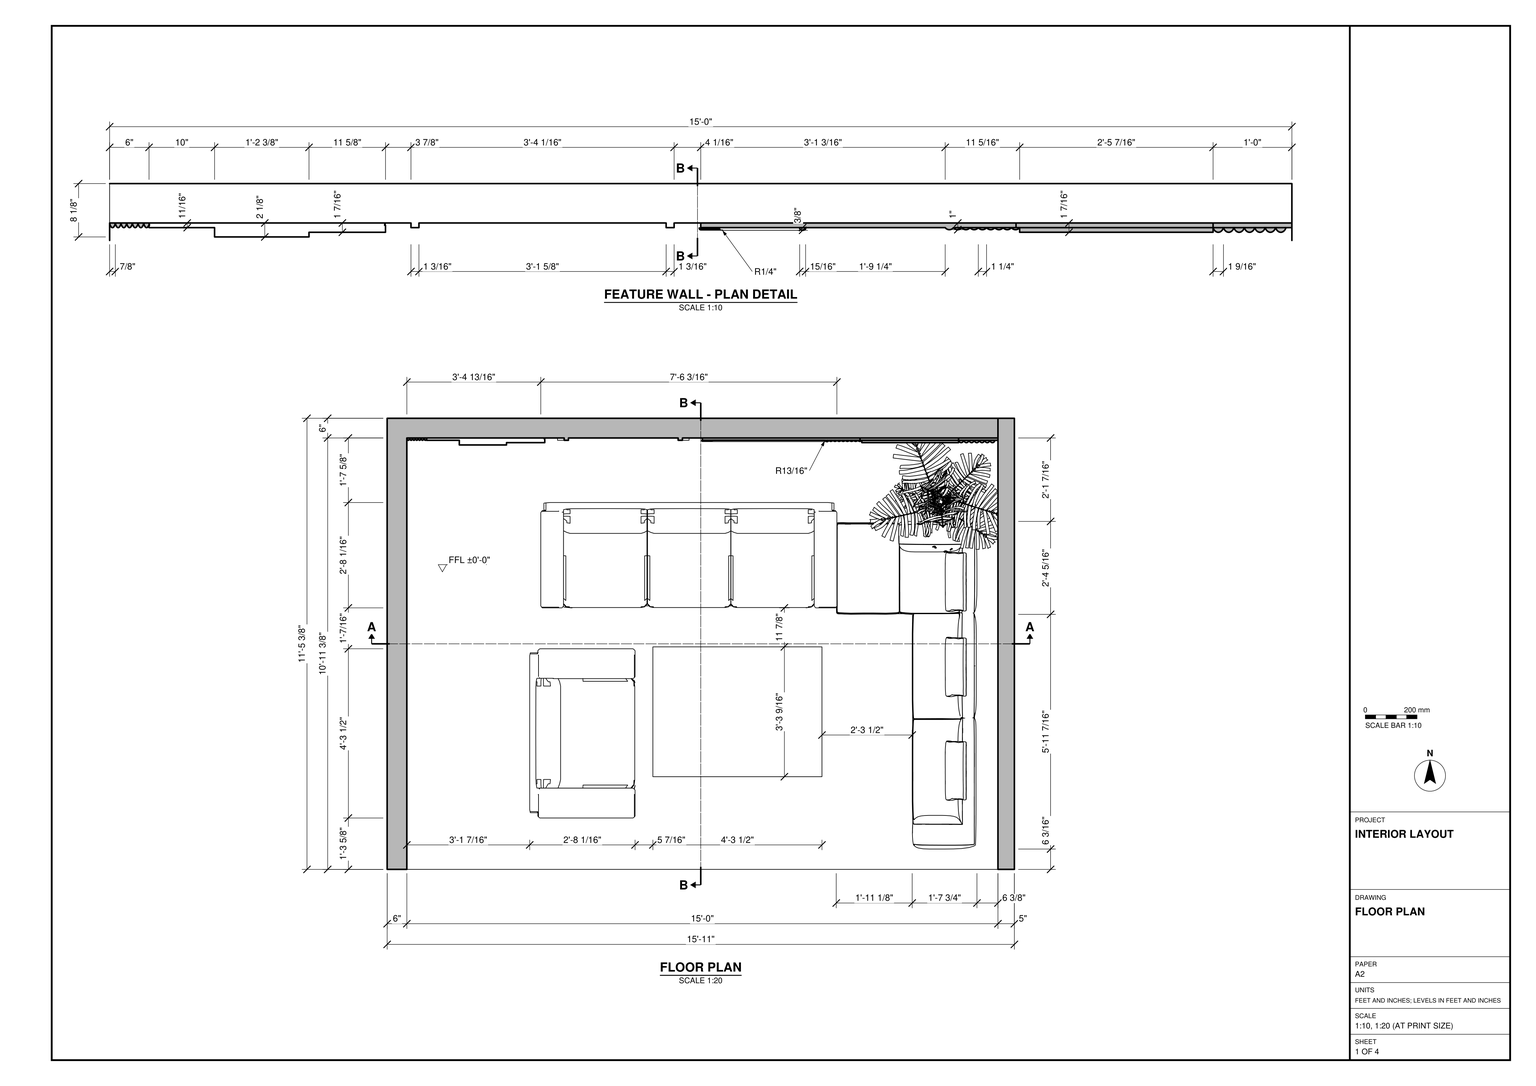
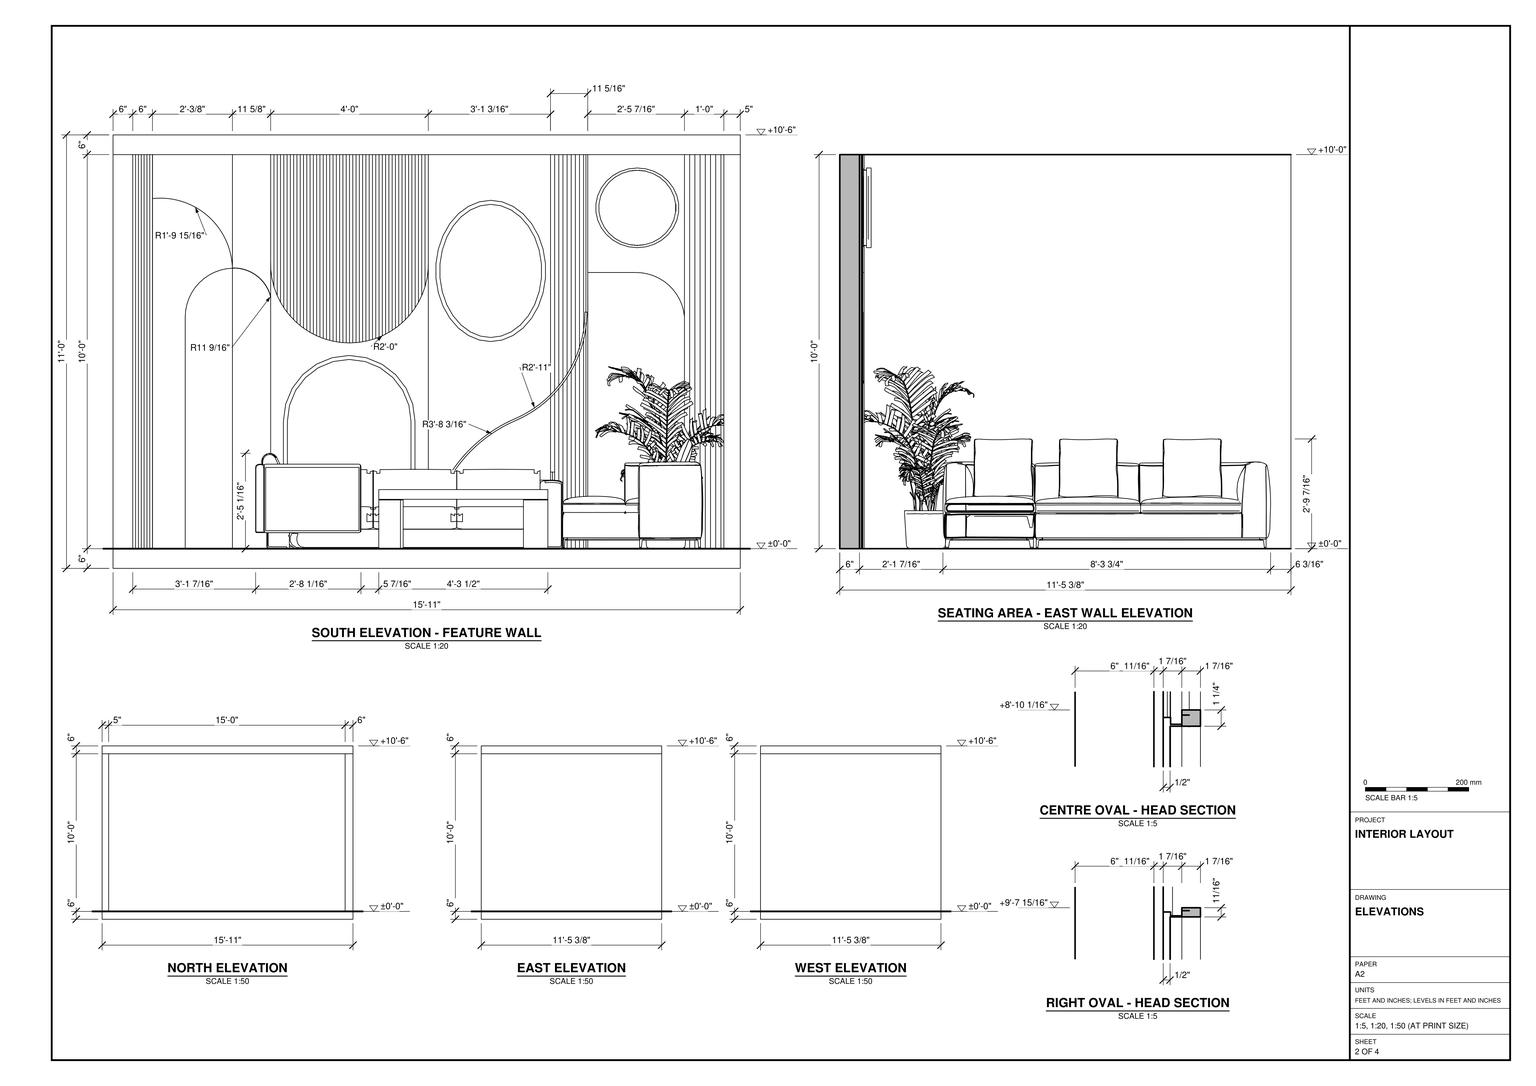
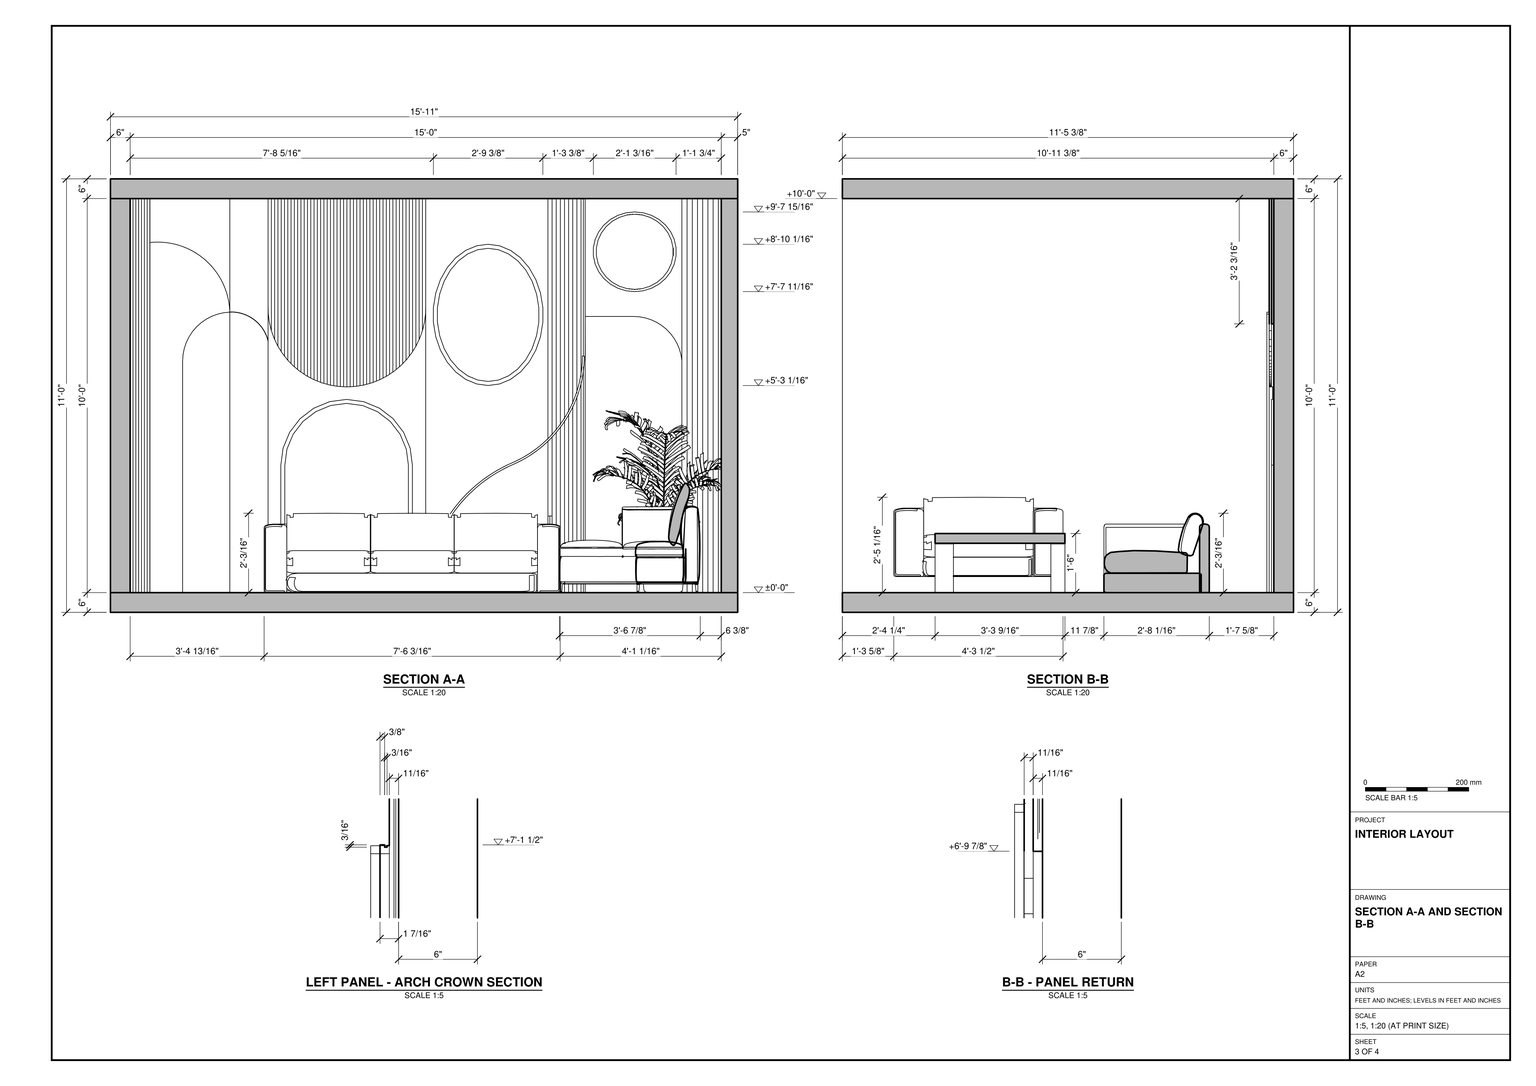
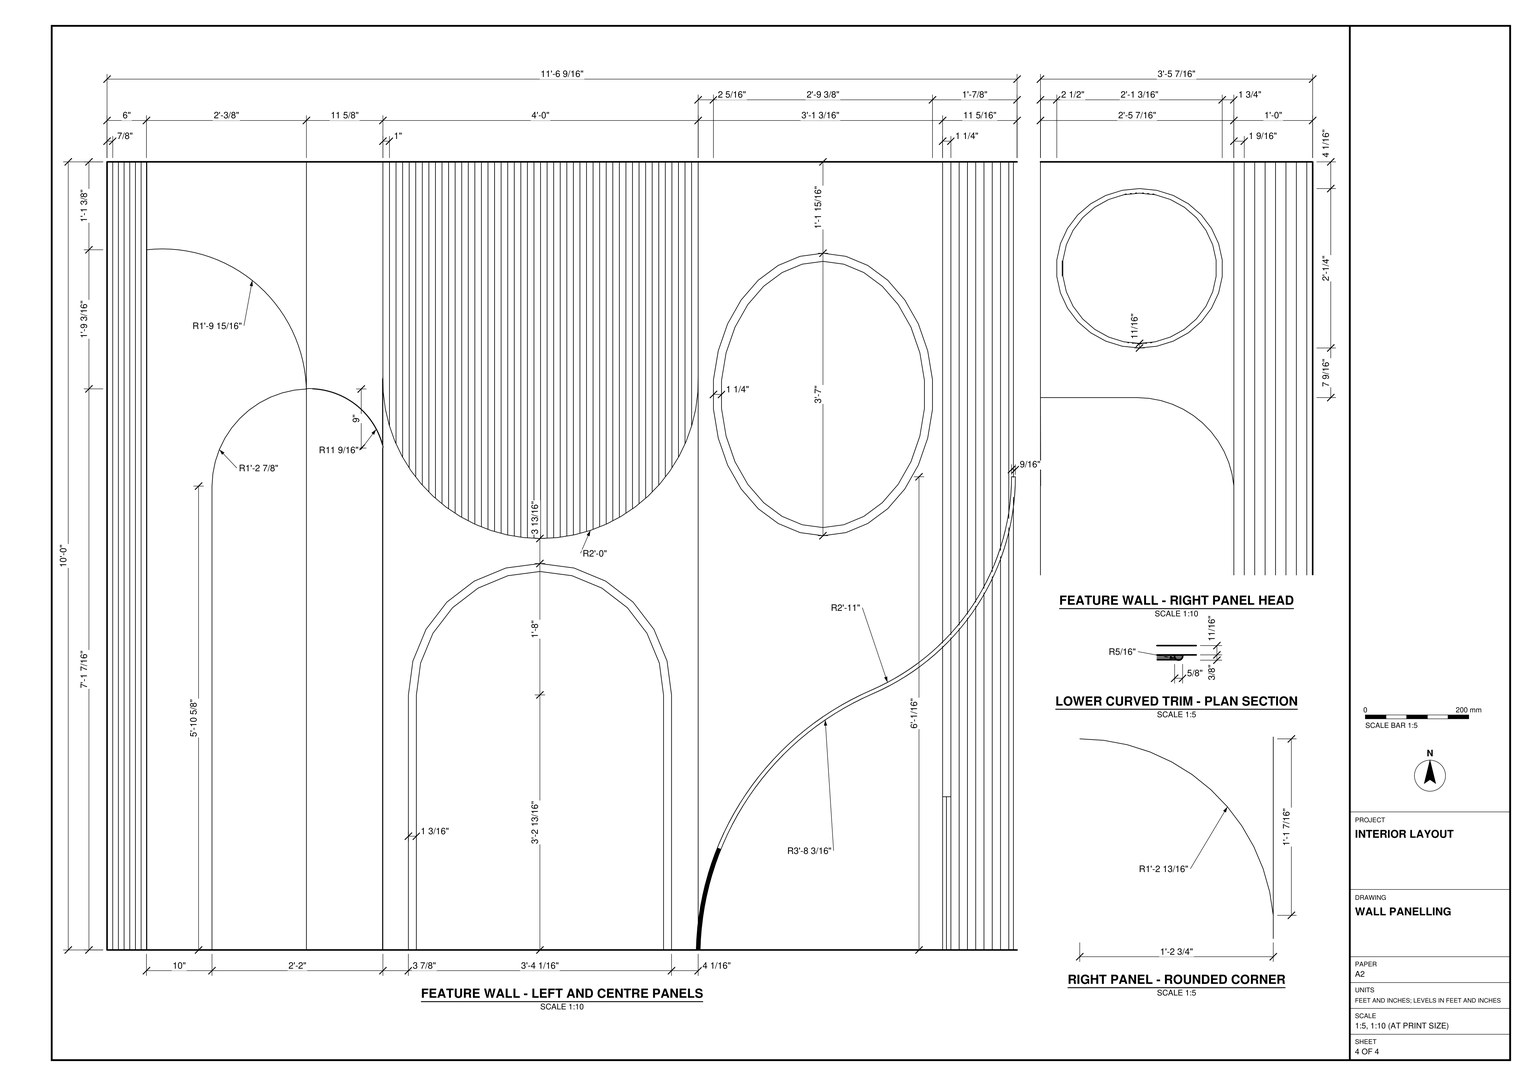
Build the seating room in SketchUp from task_files/diagram_01.pdf. Work in feet and inches. The room measures 15'-11" across the feature wall, 11'-5 3/8" from front to back and 11'-0" high overall. Use the single finished floor level of ±0'-0". Model the floor and overhead slabs with 10'-0" clear between them. Leave the front open as drawn. In plan, the left and back walls are 6" thick and the right wall is 5" thick.

Build the feature wall across the back of the room. Use the elevation to set out the ribbed fields, arched outlines, sweeping curve and two oval window units. Set the smaller oval higher and farther right than the larger one. Use the plan and section details to give the panels, ribs and rims their different projections rather than drawing a flat pattern.

Place the long sofa parallel to the feature wall, the other long seating run along the right wall and the shorter seat to the left of the rectangular coffee table. Match their footprints and clearances to the floor plan. Place the potted plant in the back right corner. Decor and loose items may be any suitable library components.

Keep the walls, slabs and each furniture or joinery piece in separate groups or components, and use components for repeated parts. Save one SketchUp model as output_files/furnished_seating_room_with_a_curved_feature_wall.skp.

# SketchUp Ruby script. Lengths in inches.
U = 1.inch
M = Sketchup.active_model
def pt(a) = Geom::Point3d.new(a.map { |v| v * U })
def face(e, loops, mat)
  f = e.add_face(loops[0].map { |a| pt(a) })
  loops[1..].each { |l| e.add_face(l.map { |a| pt(a) }).erase! }
  f.material = f.back_material = mat if mat
  f
end
# faces: each face lists its corners as indices into pts; further lists are holes
def faces(e, pts, list, mat = nil) = list.each { |f| face(e, (f[0].is_a?(Array) ? f : [f]).map { |l| l.map { |i| pts[i] } }, mat) }
# xy, xz, yz: faces in a plane at the given z, y or x. An outline is a flat list of corners, or four numbers for a rectangle; further outlines are holes
def ring(l) = l.size == 4 ? [[l[0], l[1]], [l[2], l[1]], [l[2], l[3]], [l[0], l[3]]] : l.each_slice(2).to_a
def flat(e, list, mat, &to3) = list.each { |f| face(e, (f[0].is_a?(Array) ? f : [f]).map { |l| ring(l).map { |u, v| to3.(u, v) } }, mat) }
def xy(e, z, list, mat = nil) = flat(e, list, mat) { |x, y| [x, y, z] }
def xz(e, y, list, mat = nil) = flat(e, list, mat) { |x, z| [x, y, z] }
def yz(e, x, list, mat = nil) = flat(e, list, mat) { |y, z| [x, y, z] }
def lines(e, pts, list) = list.each { |a, b| e.add_line(pt(pts[a]), pt(pts[b])) }
# prism: a flat outline (further loops are holes) pulled along v
def prism(e, loops, v, mat = nil)
  f = face(e, loops, mat); d = Geom::Vector3d.new(v.map { |x| x * U })
  f.pushpull(f.normal.samedirection?(d) ? d.length : -d.length)
end
def box(e, o, s, mat = nil) = prism(e, [[o, [o[0] + s[0], o[1], o[2]], [o[0] + s[0], o[1] + s[1], o[2]], [o[0], o[1] + s[1], o[2]]]], [0, 0, s[2]], mat)
def at(x, y, z, deg = 0) = Geom::Transformation.translation(pt([x, y, z])) * Geom::Transformation.rotation(ORIGIN, Z_AXIS, deg.degrees)
def axes(o, x, y, z) = Geom::Transformation.new([*x, 0, *y, 0, *z, 0, *pt(o).to_a, 1])
def part(name) = M.definitions.add(name)
# library, detail: a bought-in or finely detailed component or shape, given as its bounding box
def library(name, o, s) = part(name).tap { |d| box(d.entities, o, s) }
def detail(e, o, s) = box(e.add_group.entities, o, s)
def put(e, d, t, mat = nil) = e.add_instance(d, t).tap { |i| i.material = mat if mat }
def group(e, t, mat = nil) = e.add_group.tap { |g| g.transformation = t; g.material = mat if mat }.entities
root = M.entities
M.materials.add("1685 AP 8472 WILD MUSHROOM").color = [168, 160, 151]
M.materials.add("1690 AP 9522 RIVER SAND").color = [210, 197, 169]
M.materials.add("[Translucent Glass Blue]").color = [100, 149, 237]
M.materials["[Translucent Glass Blue]"].alpha = 0.5
c1 = library("michel-club1",[-34.67,-0.85,-0.13],[126.28,91.17,33.41])
c2 = library("canapele",[-55.76,140.38,0],[93.54,96.07,29.04])
c3 = library("KentiaPalm",[-22.86,-14.31,0],[47.49,43.96,59.125])
c4 = library("Group\#7",[0,-0.25,0],[6,0.25,120])
c5 = library("Group\#2",[0,-2.125,0],[36.05,2.125,120])
c6 = part("Group7\#1")
xy(c6.entities,0,[[-22,-14.24,-22.1875,-13.85,-23.04,-11.42,-23.63,-8.92,-23.95,-6.37,-24,-3.8,-24,28.67,-22,28.67]])
xy(c6.entities,0.6875,[[-22,-14.24,-22,28.67,-24,28.67,-24,-3.8,-23.95,-6.37,-23.63,-8.92,-23.04,-11.42,-22.1875,-13.85]])
yz(c6.entities,-24,[[-3.8,0,28.67,0.6875]])
yz(c6.entities,-22,[[-14.24,0,28.67,0.6875]])
c7 = part("Group8\#1")
xy(c7.entities,0,[[-21,-16.29,-21.08,-16.17,-22.1875,-13.85,-23,-11.54,-23,28.67,-21,28.67]])
xy(c7.entities,0.6875,[[-21,-16.29,-21,28.67,-23,28.67,-23,-11.54,-22.1875,-13.85,-21.08,-16.17]])
xz(c7.entities,28.67,[[-23,0,-21,0.6875]])
yz(c7.entities,-23,[[-11.54,0,28.67,0.6875]])
yz(c7.entities,-21,[[-16.29,0,28.67,0.6875]])
c8 = part("Group9\#1")
xy(c8.entities,0,[[-20,-17.91,-21.08,-16.17,-22,-14.24,-22,28.67,-20,28.67]])
xy(c8.entities,0.6875,[[-20,-17.91,-20,28.67,-22,28.67,-22,-14.24,-21.08,-16.17]])
xz(c8.entities,28.67,[[-22,0,-20,0.6875]])
yz(c8.entities,-22,[[-14.24,0,28.67,0.6875]])
yz(c8.entities,-20,[[-17.91,0,28.67,0.6875]])
c9 = part("Group10\#1")
xy(c9.entities,0,[[-19,-19.29,-19.73,-18.35,-21,-16.29,-21,28.67,-19,28.67]])
xy(c9.entities,0.6875,[[-19,-19.29,-19,28.67,-21,28.67,-21,-16.29,-19.73,-18.35]])
yz(c9.entities,-21,[[-16.29,0,28.67,0.6875]])
yz(c9.entities,-19,[[-19.29,0,28.67,0.6875]])
c10 = part("Group11\#1")
xy(c10.entities,0,[[-18,-20.54,-18.15,-20.38,-19.73,-18.35,-20,-17.91,-20,28.67,-18,28.67]])
xy(c10.entities,0.6875,[[-18,-20.54,-18,28.67,-20,28.67,-20,-17.91,-19.73,-18.35,-18.15,-20.38]])
xz(c10.entities,28.67,[[-20,0,-18,0.6875]])
yz(c10.entities,-20,[[-17.91,0,28.67,0.6875]])
yz(c10.entities,-18,[[-20.54,0,28.67,0.6875]])
c11 = part("Group12\#1")
xy(c11.entities,0,[[-17,-21.58,-18.15,-20.38,-19,-19.29,-19,28.67,-17,28.67]])
xy(c11.entities,0.6875,[[-17,-21.58,-17,28.67,-19,28.67,-19,-19.29,-18.15,-20.38]])
xz(c11.entities,28.67,[[-19,0,-17,0.6875]])
yz(c11.entities,-19,[[-19.29,0,28.67,0.6875]])
yz(c11.entities,-17,[[-21.58,0,28.67,0.6875]])
c12 = part("Group13\#1")
xy(c12.entities,0,[[-16,-22.54,-16.37,-22.23,-18,-20.54,-18,28.67,-16,28.67]])
xy(c12.entities,0.6875,[[-16,-22.54,-16,28.67,-18,28.67,-18,-20.54,-16.37,-22.23]])
yz(c12.entities,-18,[[-20.54,0,28.67,0.6875]])
yz(c12.entities,-16,[[-22.54,0,28.67,0.6875]])
c13 = part("Group14\#1")
xy(c13.entities,0,[[-15,-23.375,-16.37,-22.23,-17,-21.58,-17,28.67,-15,28.67]])
xy(c13.entities,0.6875,[[-15,-23.375,-15,28.67,-17,28.67,-17,-21.58,-16.37,-22.23]])
xz(c13.entities,28.67,[[-17,0,-15,0.6875]])
yz(c13.entities,-17,[[-21.58,0,28.67,0.6875]])
yz(c13.entities,-15,[[-23.375,0,28.67,0.6875]])
c14 = part("Group15\#1")
xy(c14.entities,0,[[-14,-24.14,-14.39,-23.88,-16,-22.54,-16,28.67,-14,28.67]])
xy(c14.entities,0.6875,[[-14,-24.14,-14,28.67,-16,28.67,-16,-22.54,-14.39,-23.88]])
xz(c14.entities,28.67,[[-16,0,-14,0.6875]])
yz(c14.entities,-16,[[-22.54,0,28.67,0.6875]])
yz(c14.entities,-14,[[-24.14,0,28.67,0.6875]])
c15 = part("Group16\#1")
xy(c15.entities,0,[[-13,-24.8125,-14.39,-23.88,-15,-23.375,-15,28.67,-13,28.67]])
xy(c15.entities,0.6875,[[-13,-24.8125,-13,28.67,-15,28.67,-15,-23.375,-14.39,-23.88]])
xz(c15.entities,28.67,[[-15,0,-13,0.6875]])
yz(c15.entities,-15,[[-23.375,0,28.67,0.6875]])
yz(c15.entities,-13,[[-24.8125,0,28.67,0.6875]])
c16 = part("Group17\#1")
xy(c16.entities,0,[[-12,-25.44,-12.26,-25.3125,-14,-24.14,-14,28.67,-12,28.67]])
xy(c16.entities,0.6875,[[-12,-25.44,-12,28.67,-14,28.67,-14,-24.14,-12.26,-25.3125]])
xz(c16.entities,28.67,[[-14,0,-12,0.6875]])
yz(c16.entities,-14,[[-24.14,0,28.67,0.6875]])
yz(c16.entities,-12,[[-25.44,0,28.67,0.6875]])
c17 = part("Group18\#1")
xy(c17.entities,0,[[-11,-25.97,-12.26,-25.3125,-13,-24.8125,-13,28.67,-11,28.67]])
xy(c17.entities,0.6875,[[-11,-25.97,-11,28.67,-13,28.67,-13,-24.8125,-12.26,-25.3125]])
xz(c17.entities,28.67,[[-13,0,-11,0.6875]])
yz(c17.entities,-13,[[-24.8125,0,28.67,0.6875]])
yz(c17.entities,-11,[[-25.97,0,28.67,0.6875]])
c18 = part("Group19\#1")
prism(c18.entities,[[[-10,28.67,0],[-10,-26.49,0],[-12,-25.44,0],[-12,28.67,0]]],[0,0,0.6875])
c19 = part("Group20\#1")
xy(c19.entities,0,[[-9,-26.89,-9.98,-26.5,-11,-25.97,-11,28.67,-9,28.67]])
xy(c19.entities,0.6875,[[-9,-26.89,-9,28.67,-11,28.67,-11,-25.97,-9.98,-26.5]])
xz(c19.entities,28.67,[[-11,0,-9,0.6875]])
yz(c19.entities,-11,[[-25.97,0,28.67,0.6875]])
yz(c19.entities,-9,[[-26.89,0,28.67,0.6875]])
c20 = part("Group21\#1")
xy(c20.entities,0,[[-8,-27.28,-9.98,-26.5,-10,-26.49,-10,28.67,-8,28.67]])
xy(c20.entities,0.6875,[[-8,-27.28,-8,28.67,-10,28.67,-10,-26.49,-9.98,-26.5]])
xz(c20.entities,28.67,[[-10,0,-8,0.6875]])
yz(c20.entities,-10,[[-26.49,0,28.67,0.6875]])
yz(c20.entities,-8,[[-27.28,0,28.67,0.6875]])
c21 = part("Group22\#1")
xy(c21.entities,0,[[-7,-27.6,-7.58,-27.44,-9,-26.89,-9,28.67,-7,28.67]])
xy(c21.entities,0.6875,[[-7,-27.6,-7,28.67,-9,28.67,-9,-26.89,-7.58,-27.44]])
xz(c21.entities,28.67,[[-9,0,-7,0.6875]])
yz(c21.entities,-9,[[-26.89,0,28.67,0.6875]])
yz(c21.entities,-7,[[-27.6,0,28.67,0.6875]])
c22 = part("Group23\#1")
xy(c22.entities,0,[[-6,-27.88,-7.58,-27.44,-8,-27.28,-8,28.67,-6,28.67]])
xy(c22.entities,0.6875,[[-6,-27.88,-6,28.67,-8,28.67,-8,-27.28,-7.58,-27.44]])
xz(c22.entities,28.67,[[-8,0,-6,0.6875]])
yz(c22.entities,-8,[[-27.28,0,28.67,0.6875]])
yz(c22.entities,-6,[[-27.88,0,28.67,0.6875]])
c23 = part("Group24\#1")
xy(c23.entities,0,[[-5,-28.14,-5.11,-28.125,-7,-27.6,-7,28.67,-5,28.67]])
xy(c23.entities,0.6875,[[-5,-28.14,-5,28.67,-7,28.67,-7,-27.6,-5.11,-28.125]])
xz(c23.entities,28.67,[[-7,0,-5,0.6875]])
yz(c23.entities,-7,[[-27.6,0,28.67,0.6875]])
yz(c23.entities,-5,[[-28.14,0,28.67,0.6875]])
c24 = part("Group25\#1")
xy(c24.entities,0,[[-4,-28.3,-5.11,-28.125,-6,-27.88,-6,28.67,-4,28.67]])
xy(c24.entities,0.6875,[[-4,-28.3,-4,28.67,-6,28.67,-6,-27.88,-5.11,-28.125]])
yz(c24.entities,-6,[[-27.88,0,28.67,0.6875]])
yz(c24.entities,-4,[[-28.3,0,28.67,0.6875]])
c25 = part("Group26\#1")
prism(c25.entities,[[[-5,-28.14,0],[-5,28.67,0],[-3,28.67,0],[-3,-28.47,0]]],[0,0,0.6875])
c26 = part("Group27\#1")
xy(c26.entities,0,[[-2,-28.57,-2.57,-28.54,-4,-28.3,-4,28.67,-2,28.67]])
xy(c26.entities,0.6875,[[-2,-28.57,-2,28.67,-4,28.67,-4,-28.3,-2.57,-28.54]])
xz(c26.entities,28.67,[[-4,0,-2,0.6875]])
yz(c26.entities,-4,[[-28.3,0,28.67,0.6875]])
yz(c26.entities,-2,[[-28.57,0,28.67,0.6875]])
c27 = part("Group28\#1")
xy(c27.entities,0,[[-1,-28.62,-2.57,-28.54,-3,-28.47,-3,28.67,-1,28.67]])
xy(c27.entities,0.6875,[[-1,-28.62,-1,28.67,-3,28.67,-3,-28.47,-2.57,-28.54]])
xz(c27.entities,28.67,[[-3,0,-1,0.6875]])
yz(c27.entities,-3,[[-28.47,0,28.67,0.6875]])
yz(c27.entities,-1,[[-28.62,0,28.67,0.6875]])
c28 = part("Group29\#1")
prism(c28.entities,[[[-2,-28.57,0],[-2,28.67,0],[0,28.67,0],[0,-28.67,0]]],[0,0,0.6875])
c29 = part("Group30\#1")
xy(c29.entities,0,[[0,-28.67,-1,-28.62,-1,28.67,1,28.67,1,-28.62]])
xy(c29.entities,0.6875,[[0,-28.67,1,-28.62,1,28.67,-1,28.67,-1,-28.62]])
xz(c29.entities,28.67,[[-1,0,1,0.6875]])
yz(c29.entities,-1,[[-28.62,0,28.67,0.6875]])
yz(c29.entities,1,[[-28.62,0,28.67,0.6875]])
c30 = part("Group31\#1")
prism(c30.entities,[[[0,-28.67,0],[0,28.67,0],[2,28.67,0],[2,-28.57,0]]],[0,0,0.6875])
c31 = part("Group32\#1")
xy(c31.entities,0,[[1,-28.62,1,28.67,3,28.67,3,-28.47,2.57,-28.54]])
xy(c31.entities,0.6875,[[1,-28.62,2.57,-28.54,3,-28.47,3,28.67,1,28.67]])
yz(c31.entities,1,[[-28.62,0,28.67,0.6875]])
yz(c31.entities,3,[[-28.47,0,28.67,0.6875]])
c32 = part("Group33\#1")
xy(c32.entities,0,[[2,-28.57,2,28.67,4,28.67,4,-28.3,2.57,-28.54]])
xy(c32.entities,0.6875,[[2,-28.57,2.57,-28.54,4,-28.3,4,28.67,2,28.67]])
xz(c32.entities,28.67,[[2,0,4,0.6875]])
yz(c32.entities,2,[[-28.57,0,28.67,0.6875]])
yz(c32.entities,4,[[-28.3,0,28.67,0.6875]])
c33 = part("Group34\#1")
prism(c33.entities,[[[3,-28.47,0],[3,28.67,0],[5,28.67,0],[5,-28.14,0]]],[0,0,0.6875])
c34 = part("Group35\#1")
xy(c34.entities,0,[[4,-28.3,4,28.67,6,28.67,6,-27.88,5.11,-28.125]])
xy(c34.entities,0.6875,[[4,-28.3,5.11,-28.125,6,-27.88,6,28.67,4,28.67]])
xz(c34.entities,28.67,[[4,0,6,0.6875]])
yz(c34.entities,4,[[-28.3,0,28.67,0.6875]])
yz(c34.entities,6,[[-27.88,0,28.67,0.6875]])
c35 = part("Group36\#1")
xy(c35.entities,0,[[5,-28.14,5,28.67,7,28.67,7,-27.6,5.11,-28.125]])
xy(c35.entities,0.6875,[[5,-28.14,5.11,-28.125,7,-27.6,7,28.67,5,28.67]])
xz(c35.entities,28.67,[[5,0,7,0.6875]])
yz(c35.entities,5,[[-28.14,0,28.67,0.6875]])
yz(c35.entities,7,[[-27.6,0,28.67,0.6875]])
c36 = part("Group37\#1")
xy(c36.entities,0,[[6,-27.88,6,28.67,8,28.67,8,-27.28,7.58,-27.44]])
xy(c36.entities,0.6875,[[6,-27.88,7.58,-27.44,8,-27.28,8,28.67,6,28.67]])
xz(c36.entities,28.67,[[6,0,8,0.6875]])
yz(c36.entities,6,[[-27.88,0,28.67,0.6875]])
yz(c36.entities,8,[[-27.28,0,28.67,0.6875]])
c37 = part("Group38\#1")
xy(c37.entities,0,[[7,-27.6,7,28.67,9,28.67,9,-26.89,7.58,-27.44]])
xy(c37.entities,0.6875,[[7,-27.6,7.58,-27.44,9,-26.89,9,28.67,7,28.67]])
xz(c37.entities,28.67,[[7,0,9,0.6875]])
yz(c37.entities,7,[[-27.6,0,28.67,0.6875]])
yz(c37.entities,9,[[-26.89,0,28.67,0.6875]])
c38 = part("Group39\#1")
xy(c38.entities,0,[[8,-27.28,8,28.67,10,28.67,10,-26.49,9.98,-26.5]])
xy(c38.entities,0.6875,[[8,-27.28,9.98,-26.5,10,-26.49,10,28.67,8,28.67]])
xz(c38.entities,28.67,[[8,0,10,0.6875]])
yz(c38.entities,8,[[-27.28,0,28.67,0.6875]])
yz(c38.entities,10,[[-26.49,0,28.67,0.6875]])
c39 = part("Group40\#1")
xy(c39.entities,0,[[9,-26.89,9,28.67,11,28.67,11,-25.97,9.98,-26.5]])
xy(c39.entities,0.6875,[[9,-26.89,9.98,-26.5,11,-25.97,11,28.67,9,28.67]])
xz(c39.entities,28.67,[[9,0,11,0.6875]])
yz(c39.entities,9,[[-26.89,0,28.67,0.6875]])
yz(c39.entities,11,[[-25.97,0,28.67,0.6875]])
c40 = part("Group41\#1")
prism(c40.entities,[[[10,-26.49,0],[10,28.67,0],[12,28.67,0],[12,-25.44,0]]],[0,0,0.6875])
c41 = part("Group42\#1")
xy(c41.entities,0,[[11,-25.97,11,28.67,13,28.67,13,-24.8125,12.26,-25.3125]])
xy(c41.entities,0.6875,[[11,-25.97,12.26,-25.3125,13,-24.8125,13,28.67,11,28.67]])
xz(c41.entities,28.67,[[11,0,13,0.6875]])
yz(c41.entities,11,[[-25.97,0,28.67,0.6875]])
yz(c41.entities,13,[[-24.8125,0,28.67,0.6875]])
c42 = part("Group43\#1")
xy(c42.entities,0,[[12,-25.44,12,28.67,14,28.67,14,-24.14,12.26,-25.3125]])
xy(c42.entities,0.6875,[[12,-25.44,12.26,-25.3125,14,-24.14,14,28.67,12,28.67]])
yz(c42.entities,12,[[-25.44,0,28.67,0.6875]])
yz(c42.entities,14,[[-24.14,0,28.67,0.6875]])
c43 = part("Group44\#1")
xy(c43.entities,0,[[13,-24.8125,13,28.67,15,28.67,15,-23.375,14.39,-23.88]])
xy(c43.entities,0.6875,[[13,-24.8125,14.39,-23.88,15,-23.375,15,28.67,13,28.67]])
xz(c43.entities,28.67,[[13,0,15,0.6875]])
yz(c43.entities,13,[[-24.8125,0,28.67,0.6875]])
yz(c43.entities,15,[[-23.375,0,28.67,0.6875]])
c44 = part("Group45\#1")
xy(c44.entities,0,[[14,-24.14,14,28.67,16,28.67,16,-22.54,14.39,-23.88]])
xy(c44.entities,0.6875,[[14,-24.14,14.39,-23.88,16,-22.54,16,28.67,14,28.67]])
xz(c44.entities,28.67,[[14,0,16,0.6875]])
yz(c44.entities,14,[[-24.14,0,28.67,0.6875]])
yz(c44.entities,16,[[-22.54,0,28.67,0.6875]])
c45 = part("Group46\#1")
xy(c45.entities,0,[[15,-23.375,15,28.67,17,28.67,17,-21.58,16.37,-22.23]])
xy(c45.entities,0.6875,[[15,-23.375,16.37,-22.23,17,-21.58,17,28.67,15,28.67]])
xz(c45.entities,28.67,[[15,0,17,0.6875]])
yz(c45.entities,15,[[-23.375,0,28.67,0.6875]])
yz(c45.entities,17,[[-21.58,0,28.67,0.6875]])
c46 = part("Group47\#1")
xy(c46.entities,0,[[16,-22.54,16,28.67,18,28.67,18,-20.54,16.37,-22.23]])
xy(c46.entities,0.6875,[[16,-22.54,16.37,-22.23,18,-20.54,18,28.67,16,28.67]])
xz(c46.entities,28.67,[[16,0,18,0.6875]])
yz(c46.entities,16,[[-22.54,0,28.67,0.6875]])
yz(c46.entities,18,[[-20.54,0,28.67,0.6875]])
c47 = part("Group48\#1")
xy(c47.entities,0,[[17,-21.58,17,28.67,19,28.67,19,-19.29,18.15,-20.38]])
xy(c47.entities,0.6875,[[17,-21.58,18.15,-20.38,19,-19.29,19,28.67,17,28.67]])
xz(c47.entities,28.67,[[17,0,19,0.6875]])
yz(c47.entities,17,[[-21.58,0,28.67,0.6875]])
yz(c47.entities,19,[[-19.29,0,28.67,0.6875]])
c48 = part("Group49\#1")
xy(c48.entities,0,[[18,-20.54,18,28.67,20,28.67,20,-17.91,19.73,-18.35,18.15,-20.38]])
xy(c48.entities,0.6875,[[18,-20.54,18.15,-20.38,19.73,-18.35,20,-17.91,20,28.67,18,28.67]])
xz(c48.entities,28.67,[[18,0,20,0.6875]])
yz(c48.entities,18,[[-20.54,0,28.67,0.6875]])
yz(c48.entities,20,[[-17.91,0,28.67,0.6875]])
c49 = part("Group50\#1")
xy(c49.entities,0,[[19,-19.29,19,28.67,21,28.67,21,-16.29,19.73,-18.35]])
xy(c49.entities,0.6875,[[19,-19.29,19.73,-18.35,21,-16.29,21,28.67,19,28.67]])
xz(c49.entities,28.67,[[19,0,21,0.6875]])
yz(c49.entities,19,[[-19.29,0,28.67,0.6875]])
yz(c49.entities,21,[[-16.29,0,28.67,0.6875]])
c50 = part("Group51\#1")
xy(c50.entities,0,[[20,-17.91,20,28.67,22,28.67,22,-14.24,21.08,-16.17]])
xy(c50.entities,0.6875,[[20,-17.91,21.08,-16.17,22,-14.24,22,28.67,20,28.67]])
xz(c50.entities,28.67,[[20,0,22,0.6875]])
yz(c50.entities,20,[[-17.91,0,28.67,0.6875]])
yz(c50.entities,22,[[-14.24,0,28.67,0.6875]])
c51 = part("Group52\#1")
xy(c51.entities,0,[[21,-16.29,21,28.67,23,28.67,23,-11.54,22.1875,-13.85,21.08,-16.17]])
xy(c51.entities,0.6875,[[21,-16.29,21.08,-16.17,22.1875,-13.85,23,-11.54,23,28.67,21,28.67]])
xz(c51.entities,28.67,[[21,0,23,0.6875]])
yz(c51.entities,21,[[-16.29,0,28.67,0.6875]])
yz(c51.entities,23,[[-11.54,0,28.67,0.6875]])
c52 = part("Group53\#1")
xy(c52.entities,0,[[22,-14.24,22,28.67,24,28.67,24,-3.8,23.95,-6.37,23.63,-8.92,23.04,-11.42,22.1875,-13.85]])
xy(c52.entities,0.6875,[[22,-14.24,22.1875,-13.85,23.04,-11.42,23.63,-8.92,23.95,-6.37,24,-3.8,24,28.67,22,28.67]])
xz(c52.entities,28.67,[[22,0,24,0.6875]])
yz(c52.entities,22,[[-14.24,0,28.67,0.6875]])
yz(c52.entities,24,[[-3.8,0,28.67,0.6875]])
c53 = part("Group5\#1")
put(c53.entities,c6,at(0,0,0))
put(c53.entities,c7,at(0,0,0))
put(c53.entities,c8,at(0,0,0))
put(c53.entities,c9,at(0,0,0))
put(c53.entities,c10,at(0,0,0))
put(c53.entities,c11,at(0,0,0))
put(c53.entities,c12,at(0,0,0))
put(c53.entities,c13,at(0,0,0))
put(c53.entities,c14,at(0,0,0))
put(c53.entities,c15,at(0,0,0))
put(c53.entities,c16,at(0,0,0))
put(c53.entities,c17,at(0,0,0))
put(c53.entities,c18,at(0,0,0))
put(c53.entities,c19,at(0,0,0))
put(c53.entities,c20,at(0,0,0))
put(c53.entities,c21,at(0,0,0))
put(c53.entities,c22,at(0,0,0))
put(c53.entities,c23,at(0,0,0))
put(c53.entities,c24,at(0,0,0))
put(c53.entities,c25,at(0,0,0))
put(c53.entities,c26,at(0,0,0))
put(c53.entities,c27,at(0,0,0))
put(c53.entities,c28,at(0,0,0))
put(c53.entities,c29,at(0,0,0))
put(c53.entities,c30,at(0,0,0))
put(c53.entities,c31,at(0,0,0))
put(c53.entities,c32,at(0,0,0))
put(c53.entities,c33,at(0,0,0))
put(c53.entities,c34,at(0,0,0))
put(c53.entities,c35,at(0,0,0))
put(c53.entities,c36,at(0,0,0))
put(c53.entities,c37,at(0,0,0))
put(c53.entities,c38,at(0,0,0))
put(c53.entities,c39,at(0,0,0))
put(c53.entities,c40,at(0,0,0))
put(c53.entities,c41,at(0,0,0))
put(c53.entities,c42,at(0,0,0))
put(c53.entities,c43,at(0,0,0))
put(c53.entities,c44,at(0,0,0))
put(c53.entities,c45,at(0,0,0))
put(c53.entities,c46,at(0,0,0))
put(c53.entities,c47,at(0,0,0))
put(c53.entities,c48,at(0,0,0))
put(c53.entities,c49,at(0,0,0))
put(c53.entities,c50,at(0,0,0))
put(c53.entities,c51,at(0,0,0))
put(c53.entities,c52,at(0,0,0))
c54 = library("Group\#3",[0,-0.25,0],[6,0.25,120])
c55 = library("Group\#4",[-0.3,-3.54,-0.01],[76.53,3.54,120.01])
put(root,c1,axes([137.15,78.57,0.13],[0,-0.79,0],[0.47,0,0],[0,0,1]))
put(root,c2,at(99.18,-124.73,0))
put(root,c3,at(167.96,107.73,0))
g1 = group(root,at(0,0,-6))
box(g1,[0,0,0],[191,137.375,6])
g2 = group(root,at(6,137.375,0))
xy(g2,0,[[-6,-137.375,0,0],[180,-137.375,185,0],[45.88,-6.71,45.88,-6,0,-6,0,0,180,0,180,-6,85.94,-6,85.94,-6.71,84.73,-6.71,84.73,-6,47.09,-6,47.09,-6.71],[138,-6.71,168,-6]])
xy(g2,120,[[-6,-137.375,0,-137.375,0,-6,180,-6,180,0,-6,0],[180,-137.375,185,0],[42,-7.4,43,-6.71],[42,-6.71,90,-6],[138,-6.71,168,-6]])
xz(g2,-137.375,[[-6,0,0,120],[180,0,185,120]])
xz(g2,-6.71,[[45.88,0,47.09,0,47.09,38.8125,47.74,43.68,49.61,48.22,52.61,52.12,56.5,55.11,61.04,56.99,65.91,57.63,70.78,56.99,75.32,55.11,79.22,52.12,82.21,48.22,84.09,43.68,84.73,38.8125,84.73,0,85.94,0,85.94,38.8125,85.26,44,83.26,48.83,80.08,52.98,75.93,56.16,71.1,58.16,65.91,58.84,60.73,58.16,55.9,56.16,51.75,52.98,48.5625,48.83,46.5625,44,45.88,38.8125],[138,0,138.55,0,138.55,84.11,153.28,84.11,155.09,83.99,156.89,83.66,158.62,83.11,160.28,82.34,161.82,81.38,163.24,80.24,164.51,78.93,165.61,77.48,166.52,75.9,167.23,74.22,167.72,72.47,168,70.67,168,120,138,120]],"1690 AP 9522 RIVER SAND")
xz(g2,-6,[[0,0,42,120],[138,0,168,120],[66,62.65,63.43,62.79,60.89,63.2,58.42,63.88,56.02,64.82,53.74,66.02,51.61,67.44,49.63,69.09,47.85,70.94,46.27,72.97,44.92,75.16,43.8125,77.48,42.96,79.91,42.37,82.41,42.05,84.96,42,87.53,42,120,90,120,90,87.53,89.95,84.96,89.63,82.41,89.04,79.91,88.1875,77.48,87.08,75.16,85.73,72.97,84.15,70.94,82.37,69.09,80.39,67.44,78.26,66.02,75.98,64.82,73.58,63.88,71.11,63.2,68.57,62.79]])
xz(g2,-6,[[47.09,0,84.73,0,84.73,38.8125,84.09,43.68,82.21,48.22,79.22,52.12,75.32,55.11,70.78,56.99,65.91,57.63,61.04,56.99,56.5,55.11,52.61,52.12,49.61,48.22,47.74,43.68,47.09,38.8125]],"1685 AP 8472 WILD MUSHROOM")
xz(g2,-6,[[42,0,45.88,0,45.88,38.8125,46.5625,44,48.5625,48.83,51.75,52.98,55.9,56.16,60.73,58.16,65.91,58.84,71.1,58.16,75.93,56.16,80.08,52.98,83.26,48.83,85.26,44,85.94,38.8125,85.94,0,90,0,90,87.53,89.95,84.96,89.63,82.41,89.04,79.91,88.1875,77.48,87.08,75.16,85.73,72.97,84.15,70.94,82.37,69.09,80.39,67.44,78.26,66.02,75.98,64.82,73.58,63.88,71.11,63.2,68.57,62.79,66,62.65,63.43,62.79,60.89,63.2,58.42,63.88,56.02,64.82,53.74,66.02,51.61,67.44,49.63,69.09,47.85,70.94,46.27,72.97,44.92,75.16,43.8125,77.48,42.96,79.91,42.37,82.41,42.05,84.96,42,87.53]],"1690 AP 9522 RIVER SAND")
xz(g2,0,[[-6,0,0,120],[0,0,180,120],[180,0,185,120]])
yz(g2,-6,[[-137.375,0,0,120]])
yz(g2,0,[[-137.375,0,-6,120]])
yz(g2,42,[[-6.71,87.53,-6,120]])
yz(g2,45.88,[[-6.71,0,-6,38.8125]])
yz(g2,47.09,[[-6.71,0,-6,38.8125]])
yz(g2,84.73,[[-6.71,0,-6,38.8125]])
yz(g2,85.94,[[-6.71,0,-6,38.8125]])
yz(g2,90,[[-6.71,87.53,-6,120]])
yz(g2,138,[[-6.71,0,-6,120]])
yz(g2,168,[[-6.71,0,-6,120]])
yz(g2,180,[[-137.375,0,0,120]])
yz(g2,185,[[-137.375,0,0,120]])
p = [[46.5625,-6,44],[45.88,-6,38.8125],[45.88,-6.71,38.8125],[46.5625,-6.71,44],[47.74,-6.71,43.68],[47.09,-6.71,38.8125],
  [47.09,-6,38.8125],[47.74,-6,43.68],[84.73,-6.71,38.8125],[84.09,-6.71,43.68],[84.09,-6,43.68],[84.73,-6,38.8125],
  [85.94,-6,38.8125],[85.26,-6,44],[85.26,-6.71,44],[85.94,-6.71,38.8125],[49.61,-6.71,48.22],[49.61,-6,48.22],
  [82.21,-6.71,48.22],[82.21,-6,48.22],[48.5625,-6,48.83],[48.5625,-6.71,48.83],[83.26,-6,48.83],[83.26,-6.71,48.83],
  [52.61,-6.71,52.12],[52.61,-6,52.12],[79.22,-6.71,52.12],[79.22,-6,52.12],[51.75,-6,52.98],[51.75,-6.71,52.98],
  [80.08,-6,52.98],[80.08,-6.71,52.98],[56.5,-6.71,55.11],[56.5,-6,55.11],[75.32,-6.71,55.11],[75.32,-6,55.11],
  [55.9,-6,56.16],[55.9,-6.71,56.16],[75.93,-6,56.16],[75.93,-6.71,56.16],[61.04,-6.71,56.99],[61.04,-6,56.99],
  [70.78,-6.71,56.99],[70.78,-6,56.99],[60.73,-6,58.16],[60.73,-6.71,58.16],[71.1,-6,58.16],[71.1,-6.71,58.16],
  [65.91,-6.71,57.63],[65.91,-6,57.63],[65.91,-6,58.84],[65.91,-6.71,58.84],[63.43,-6,62.79],[66,-6,62.65],
  [66,-6.71,62.65],[63.43,-6.71,62.79],[68.57,-6,62.79],[68.57,-6.71,62.79],[60.89,-6,63.2],[60.89,-6.71,63.2],
  [71.11,-6,63.2],[71.11,-6.71,63.2],[58.42,-6,63.88],[58.42,-6.71,63.88],[73.58,-6,63.88],[73.58,-6.71,63.88],
  [56.02,-6,64.82],[56.02,-6.71,64.82],[75.98,-6,64.82],[75.98,-6.71,64.82],[53.74,-6,66.02],[53.74,-6.71,66.02],
  [78.26,-6,66.02],[78.26,-6.71,66.02],[51.61,-6,67.44],[51.61,-6.71,67.44],[80.39,-6,67.44],[80.39,-6.71,67.44],
  [49.63,-6,69.09],[49.63,-6.71,69.09],[82.37,-6,69.09],[82.37,-6.71,69.09],[47.85,-6,70.94],[47.85,-6.71,70.94],
  [84.15,-6,70.94],[84.15,-6.71,70.94],[46.27,-6,72.97],[46.27,-6.71,72.97],[85.73,-6,72.97],[85.73,-6.71,72.97],
  [44.92,-6,75.16],[44.92,-6.71,75.16],[87.08,-6,75.16],[87.08,-6.71,75.16],[43.8125,-6,77.48],[43.8125,-6.71,77.48],
  [88.1875,-6,77.48],[88.1875,-6.71,77.48],[42.96,-6,79.91],[42.96,-6.71,79.91],[89.04,-6,79.91],[89.04,-6.71,79.91],
  [42.37,-6,82.41],[42.37,-6.71,82.41],[89.63,-6,82.41],[89.63,-6.71,82.41],[42.05,-6,84.96],[42.05,-6.71,84.96],
  [89.95,-6,84.96],[89.95,-6.71,84.96],[42,-6,87.53],[42,-6.71,87.53],[90,-6,87.53],[90,-6.71,87.53],
  [138.55,-6.71,84.11],[138.58,-6.71,70.67]]
faces(g2,p,[[0,1,2,3],[12,13,14,15],[20,0,3,21],[13,22,23,14],[28,20,21,29],[22,30,31,23],[36,28,29,37],[30,38,39,31],
  [44,36,37,45],[38,46,47,39],[50,44,45,51],[46,50,51,47]],"1690 AP 9522 RIVER SAND")
faces(g2,p,[[4,5,6,7],[8,9,10,11],[16,4,7,17],[9,18,19,10],[24,16,17,25],[18,26,27,19],[32,24,25,33],[26,34,35,27],
  [40,32,33,41],[34,42,43,35],[48,40,41,49],[42,48,49,43],[52,53,54,55],[53,56,57,54],[58,52,55,59],[56,60,61,57],
  [62,58,59,63],[60,64,65,61],[66,62,63,67],[64,68,69,65],[70,66,67,71],[68,72,73,69],[74,70,71,75],[72,76,77,73],
  [78,74,75,79],[76,80,81,77],[82,78,79,83],[80,84,85,81],[86,82,83,87],[84,88,89,85],[90,86,87,91],[88,92,93,89],
  [94,90,91,95],[92,96,97,93],[98,94,95,99],[96,100,101,97],[102,98,99,103],[100,104,105,101],[106,102,103,107],[104,108,109,105],
  [110,106,107,111],[108,112,113,109]])
lines(g2,p,[[114,115]])
put(g2,c4,axes([0,-6,0],[1.09,0,0],[0,2.83465,0],[0,0,1]),"1690 AP 9522 RIVER SAND")
put(g2,c5,at(6,-6,0),"1685 AP 8472 WILD MUSHROOM")
put(g2,c53,axes([66,-6.71,91.33],[1,0,0],[0,0,1],[0,-1,0]),"1690 AP 9522 RIVER SAND")
g3 = group(g2,at(168,-6,0))
box(g3,[0,-0.71,0],[12,0.71,120])
put(g2,c54,axes([168,-6.71,0],[2,0,0],[0,2.83465,0],[0,0,1]))
put(g2,c55,at(90,-6,0),"[Translucent Glass Blue]")
g4 = group(g2,at(138.55,-6.71,0))
xy(g4,0,[[0,-0.71,29.45,0]])
xy(g4,84.11,[[0,-0.71,14.72,0]])
xz(g4,-0.71,[[0,0,29.45,0,29.45,70.67,29.17,72.47,28.67,74.22,27.96,75.9,27.06,77.48,25.96,78.93,24.69,80.24,23.27,81.38,21.72,82.34,20.07,83.11,18.33,83.66,16.54,83.99,14.72,84.11,0,84.11]],"1690 AP 9522 RIVER SAND")
xz(g4,0,[[0,0,0,84.11,14.72,84.11,16.54,83.99,18.33,83.66,20.07,83.11,21.72,82.34,23.27,81.38,24.69,80.24,25.96,78.93,27.06,77.48,27.96,75.9,28.67,74.22,29.17,72.47,29.45,70.67,29.45,0]])
yz(g4,0,[[-0.71,0,0,84.11]])
yz(g4,29.45,[[-0.71,0,0,70.67]])
p = [[29.45,0,70.67],[29.17,0,72.47],[29.17,-0.71,72.47],[29.45,-0.71,70.67],[28.67,0,74.22],[28.67,-0.71,74.22],
  [27.96,0,75.9],[27.96,-0.71,75.9],[27.06,0,77.48],[27.06,-0.71,77.48],[25.96,0,78.93],[25.96,-0.71,78.93],
  [24.69,0,80.24],[24.69,-0.71,80.24],[23.27,0,81.38],[23.27,-0.71,81.38],[21.72,0,82.34],[21.72,-0.71,82.34],
  [20.07,0,83.11],[20.07,-0.71,83.11],[18.33,0,83.66],[18.33,-0.71,83.66],[16.54,0,83.99],[16.54,-0.71,83.99],
  [14.72,0,84.11],[14.72,-0.71,84.11]]
faces(g4,p,[[0,1,2,3],[1,4,5,2],[4,6,7,5],[6,8,9,7],[8,10,11,9],[10,12,13,11],[12,14,15,13],[14,16,17,15],
  [16,18,19,17],[18,20,21,19],[20,22,23,21],[22,24,25,23]])
g5 = group(root,at(0,0,120))
xy(g5,0,[[0,0,0,137.375,191,137.375,191,0,186,0,186,130.67,6,130.67,6,0],[6,0,186,130.67]])
xy(g5,6,[[0,0,191,137.375]])
xz(g5,0,[[0,0,191,6]])
xz(g5,137.375,[[0,0,191,6]])
yz(g5,0,[[0,0,137.375,6]])
yz(g5,191,[[0,0,137.375,6]])
